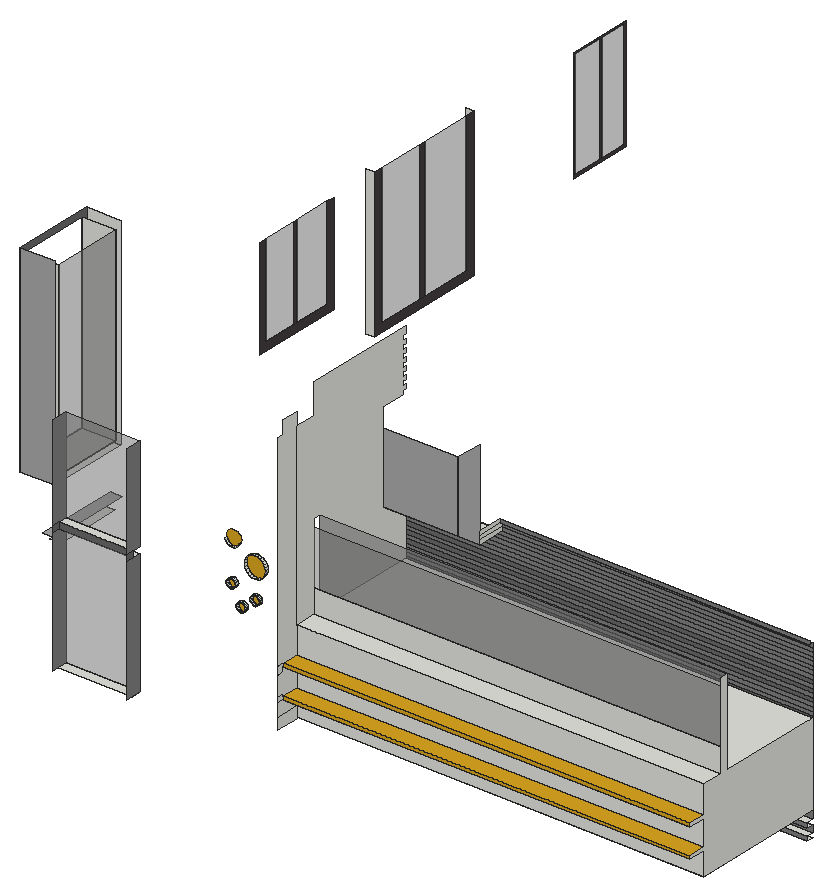
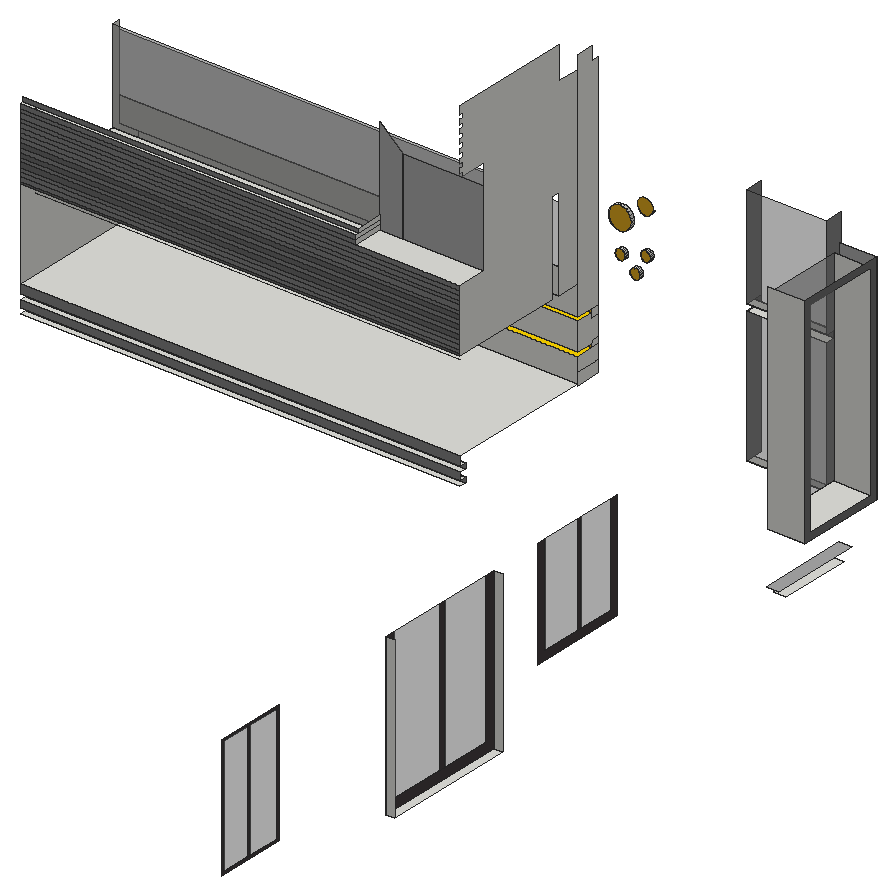
# SketchUp Ruby script. Lengths in inches.
U = 1.inch
M = Sketchup.active_model
def pt(a) = Geom::Point3d.new(a.map { |v| v * U })
def face(e, loops, mat)
  f = e.add_face(loops[0].map { |a| pt(a) })
  loops[1..].each { |l| e.add_face(l.map { |a| pt(a) }).erase! }
  f.material = f.back_material = mat if mat
  f
end
# faces: each face lists its corners as indices into pts; further lists are holes
def faces(e, pts, list, mat = nil) = list.each { |f| face(e, (f[0].is_a?(Array) ? f : [f]).map { |l| l.map { |i| pts[i] } }, mat) }
# xy, xz, yz: faces in a plane at the given z, y or x. An outline is a flat list of corners, or four numbers for a rectangle; further outlines are holes
def ring(l) = l.size == 4 ? [[l[0], l[1]], [l[2], l[1]], [l[2], l[3]], [l[0], l[3]]] : l.each_slice(2).to_a
def flat(e, list, mat, &to3) = list.each { |f| face(e, (f[0].is_a?(Array) ? f : [f]).map { |l| ring(l).map { |u, v| to3.(u, v) } }, mat) }
def xy(e, z, list, mat = nil) = flat(e, list, mat) { |x, y| [x, y, z] }
def xz(e, y, list, mat = nil) = flat(e, list, mat) { |x, z| [x, y, z] }
def yz(e, x, list, mat = nil) = flat(e, list, mat) { |y, z| [x, y, z] }
def lines(e, pts, list) = list.each { |a, b| e.add_line(pt(pts[a]), pt(pts[b])) }
# prism: a flat outline (further loops are holes) pulled along v
def prism(e, loops, v, mat = nil)
  f = face(e, loops, mat); d = Geom::Vector3d.new(v.map { |x| x * U })
  f.pushpull(f.normal.samedirection?(d) ? d.length : -d.length)
end
def box(e, o, s, mat = nil) = prism(e, [[o, [o[0] + s[0], o[1], o[2]], [o[0] + s[0], o[1] + s[1], o[2]], [o[0], o[1] + s[1], o[2]]]], [0, 0, s[2]], mat)
def at(x, y, z, deg = 0) = Geom::Transformation.translation(pt([x, y, z])) * Geom::Transformation.rotation(ORIGIN, Z_AXIS, deg.degrees)
def axes(o, x, y, z) = Geom::Transformation.new([*x, 0, *y, 0, *z, 0, *pt(o).to_a, 1])
def part(name) = M.definitions.add(name)
# library, detail: a bought-in or finely detailed component or shape, given as its bounding box
def library(name, o, s) = part(name).tap { |d| box(d.entities, o, s) }
def detail(e, o, s) = box(e.add_group.entities, o, s)
def put(e, d, t, mat = nil) = e.add_instance(d, t).tap { |i| i.material = mat if mat }
def group(e, t, mat = nil) = e.add_group.tap { |g| g.transformation = t; g.material = mat if mat }.entities
root = M.entities
M.materials.add("[0045_Goldenrod]").color = [218, 165, 32]
M.materials.add("[0046_Gold]").color = [255, 215, 0]
M.materials.add("[0132_LightGray]").color = [169, 169, 169]
M.materials.add("[0133_Gray]").color = [128, 128, 128]
M.materials.add("[0134_DimGray]").color = [105, 105, 105]
M.materials.add("[Asphalt New]").color = [67, 60, 62]
M.materials.add("[Translucent Glass Gray]").color = [128, 128, 128]
M.materials["[Translucent Glass Gray]"].alpha = 0.5
xy(root,66.12,[[241.18,136.58,366.5,138.52]])
xy(root,67.4375,[[174.32,88.83,197.1,91.46]])
xy(root,67.625,[[241.18,136.58,366.5,138.52]])
xy(root,69.69,[[241.18,136.58,366.5,138.52]])
xy(root,71.22,[[241.18,136.58,366.5,138.52]])
xy(root,73.87,[[241.18,96.65,366.5,138.52]])
xy(root,75.79,[[142.375,125.2,145.875,145.94]])
xy(root,78.39,[[142.375,122.6,145.875,148.54]],"[0132_LightGray]")
xy(root,79.7,[[143.25,245.77,145.875,284.1]])
xy(root,80.87,[[241.18,91.46,366.5,96.65]],"[0046_Gold]")
xy(root,81.9375,[[241.18,91.46,366.5,96.65]],"[0045_Goldenrod]")
xy(root,89.85,[[241.18,91.46,366.5,96.65]],"[0046_Gold]")
xy(root,90.9375,[[241.18,91.46,366.5,96.65]],"[0045_Goldenrod]")
xy(root,92.89,[[135.375,122.53,145.875,148.03]])
xy(root,94.72,[[135.375,124.36,145.875,146.21]])
xy(root,99.3125,[[241.18,96.65,366.5,103.28],[241.18,105.72,366.5,138.52]])
xy(root,105.6875,[[174.32,88.83,197.1,91.46]])
xy(root,107.62,[[174.32,88.83,197.1,91.46]])
xy(root,117.32,[[264.37,129.83,264.37,129.9,241.18,129.9,241.18,138.52,271.01,138.52,271.01,129.83]])
xy(root,119.82,[[271.01,137.46,362.29,138.52],[362.29,137.46,366.5,138.52]])
xz(root,88.83,[[174.32,105.6875,197.1,107.62]],"[0134_DimGray]")
xz(root,90.15,[[227.13,118.98,227.72,119.06,228.26,119.28,228.72,119.64,229.08,120.11,229.31,120.65,229.38,121.23,229.31,121.8125,229.08,122.36,228.72,122.82,228.26,123.18,227.72,123.4,227.13,123.48,226.55,123.4,226.01,123.18,225.54,122.82,225.19,122.36,224.96,121.8125,224.88,121.23,224.96,120.65,225.19,120.11,225.54,119.64,226.01,119.28,226.55,119.06]],"[0045_Goldenrod]")
xz(root,90.27,[[234.1875,112.62,235.03,112.73,235.8125,113.05,236.49,113.57,237,114.24,237.33,115.02,237.4375,115.87,237.33,116.71,237,117.49,236.49,118.16,235.8125,118.68,235.03,119.01,234.1875,119.12,233.35,119.01,232.5625,118.68,231.89,118.16,231.375,117.49,231.05,116.71,230.9375,115.87,231.05,115.02,231.375,114.24,231.89,113.57,232.5625,113.05,233.35,112.73]],"[0045_Goldenrod]")
xz(root,90.33,[[234.12,105.15,234.49,105.2,234.84,105.34,235.13,105.57,235.36,105.87,235.5,106.21,235.55,106.59,235.5,106.96,235.36,107.3,235.13,107.6,234.84,107.83,234.49,107.97,234.12,108.02,233.74,107.97,233.4,107.83,233.1,107.6,232.87,107.3,232.73,106.96,232.68,106.59,232.73,106.21,232.87,105.87,233.1,105.57,233.4,105.34,233.74,105.2]],"[0045_Goldenrod]")
xz(root,90.4,[[229.8,101.75,230.17,101.79,230.51,101.9375,230.8125,102.17,231.04,102.46,231.18,102.8125,231.23,103.18,231.18,103.55,231.04,103.9,230.8125,104.2,230.51,104.43,230.17,104.57,229.8,104.62,229.42,104.57,229.08,104.43,228.78,104.2,228.55,103.9,228.41,103.55,228.36,103.18,228.41,102.8125,228.55,102.46,228.78,102.17,229.08,101.9375,229.42,101.79]],"[0045_Goldenrod]")
xz(root,90.46,[[226.74,107.31,227.11,107.35,227.46,107.5,227.75,107.73,227.98,108.02,228.125,108.37,228.18,108.74,228.125,109.12,227.98,109.46,227.75,109.76,227.46,109.99,227.11,110.13,226.74,110.18,226.37,110.13,226.02,109.99,225.72,109.76,225.49,109.46,225.35,109.12,225.3,108.74,225.35,108.37,225.49,108.02,225.72,107.73,226.02,107.5,226.37,107.35]],"[0045_Goldenrod]")
xz(root,91.46,[[241.18,80.87,366.5,81.9375],[241.18,89.85,366.5,90.9375]],"[0045_Goldenrod]")
xz(root,91.46,[[174.32,67.4375,197.1,105.6875],[174.32,107.62,197.1,136.72]],"[Translucent Glass Gray]")
xz(root,96.65,[[241.18,73.87,366.5,80.87],[241.18,81.9375,366.5,89.85],[241.18,90.9375,366.5,99.3125]])
xz(root,103.28,[[241.18,99.3125,366.5,106.59]])
xz(root,103.28,[[241.18,106.59,366.5,123.39]],"[Translucent Glass Gray]")
xz(root,105.72,[[241.18,99.3125,366.5,125.6875]],"[Translucent Glass Gray]")
xz(root,122.53,[[135.375,92.89,145.875,154.77]],"[0132_LightGray]")
xz(root,124.36,[[135.375,94.72,145.875,152.9375]])
xz(root,129.83,[[264.37,117.32,271.01,117.32,271.01,144.82,264.37,139.03]],"[0132_LightGray]")
xz(root,129.9,[[241.18,117.32,264.37,139.03]],"[0132_LightGray]")
xz(root,136.58,[[241.18,66.12,366.5,67.625],[241.18,69.69,366.5,71.22]],"[0133_Gray]")
xz(root,137.46,[[271.01,119.82,366.5,121]],"[0133_Gray]")
xz(root,138.52,[[241.18,67.625,366.5,69.69],[241.18,71.22,366.5,73.87],[241.18,99.82,366.5,101],[241.18,101,366.5,102.32],[241.18,102.32,366.5,103.5],
  [241.18,104.82,366.5,106],[241.18,107.32,366.5,108.5],[241.18,109.82,366.5,111],[241.18,111,366.5,112.32],[241.18,112.32,366.5,113.5],
  [241.18,113.5,366.5,114.82],[241.18,114.82,366.5,116],[241.18,116,366.5,117.32],[271.01,117.32,366.5,118.5],[271.01,118.5,366.5,119.82]],"[0133_Gray]")
xz(root,138.52,[[241.18,99.3125,366.5,99.82],[241.18,103.5,366.5,104.82],[241.18,106,366.5,107.32],[241.18,108.5,366.5,109.82]],"[0134_DimGray]")
xz(root,146.21,[[135.375,94.72,145.875,152.9375]])
xz(root,148.03,[[135.375,92.89,145.875,154.77]])
xz(root,245.77,[[143.25,79.7,145.875,125.14]])
xz(root,284.1,[[143.25,79.7,145.875,125.14]])
yz(root,135.375,[[[122.53,92.89,148.03,154.77],[124.36,94.72,146.21,152.9375]]],"[0134_DimGray]")
yz(root,145.875,[[245.77,79.7,245.77,125.14,248.5,125.14,248.5,82.42,281.37,82.42,281.37,125.14,284.1,125.14,284.1,79.7],[263.24,82.42,264.94,125.14],[[322.32,89.76,342.57,124.57],[323.02,90.45,341.875,123.87]],[332.45,90.45,333.16,123.87],[201.67,94.21,201.67,125.14,204.1,125.14,204.1,96.64,227.54,96.64,227.54,125.14,229.97,125.14,229.97,94.21],
  [214.54,96.64,215.82,125.14]],"[Asphalt New]")
yz(root,145.875,[[248.5,82.42,263.24,125.14],[264.94,82.42,281.37,125.14],[323.02,90.45,332.45,123.87],[333.16,90.45,341.875,123.87],[124.36,94.72,146.21,152.9375],
  [204.1,96.64,214.54,125.14],[215.82,96.64,227.54,125.14]],"[Translucent Glass Gray]")
yz(root,174.32,[[86.4,67.4375,91.46,105.6875],[86.4,107.62,91.46,136.72]],"[0133_Gray]")
yz(root,174.32,[[86.4,105.6875,88.83,107.62]],"[0134_DimGray]")
yz(root,197.1,[[86.4,67.4375,91.46,105.6875],[86.4,107.62,91.46,136.72]],"[0133_Gray]")
yz(root,197.1,[[86.4,105.6875,88.83,107.62]],"[0134_DimGray]")
yz(root,241.18,[[89.33,73.43,96.65,76.93],[89.33,76.93,96.65,80.87],[89.33,80.87,91.46,82.5625],[91.46,81.9375,96.65,81.9375,96.65,89.85,91.46,89.85,91.46,88.48,89.33,88.48,89.33,82.5625,91.46,82.5625],[89.33,88.48,91.46,90.9375],
  [89.33,90.9375,96.65,90.9375,96.65,158,91.46,158,91.46,154.0625,89.33,154.0625],[96.65,99.3125,103.28,99.3125,103.28,125.6875,105.72,125.6875,105.72,99.3125,138.52,99.3125,138.52,117.32,129.9,117.32,129.9,144.82,137.46,144.82,137.46,146,138.52,146,138.52,147.32,137.46,147.32,137.46,148.5,138.52,148.5,138.52,149.82,137.46,149.82,137.46,151,138.52,151,138.52,152.32,137.46,152.32,137.46,153.5,138.52,153.5,138.52,154.82,137.46,154.82,137.46,156,138.52,156,138.52,157.32,137.46,157.32,137.46,158.5,138.52,158.5,138.52,159.82,137.46,159.82,137.46,161.04,138.52,161.04,138.52,163.35,103.2,163.35,103.2,154.0625,96.65,154.0625]])
yz(root,264.37,[[129.83,117.32,129.9,139.03]])
yz(root,271.01,[[129.83,117.32,138.52,118.5],[129.83,118.5,138.52,119.82],[129.83,119.82,137.46,121]])
yz(root,366.5,[[96.65,73.87,138.52,73.87,138.52,99.3125,105.72,99.3125,105.72,125.6875,103.28,125.6875,103.28,99.3125,96.65,99.3125,96.65,90.9375,91.46,90.9375,91.46,89.85,96.65,89.85,96.65,81.9375,91.46,81.9375,91.46,80.87,96.65,80.87]])
p = [[229.42,89.33,101.79],[229.8,89.33,101.75],[229.8,90.4,101.75],[229.42,90.4,101.79],[230.17,89.33,101.79],[230.17,90.4,101.79],
  [229.08,89.33,101.9375],[229.08,90.4,101.9375],[230.51,89.33,101.9375],[230.51,90.4,101.9375],[228.78,89.33,102.17],[228.78,90.4,102.17],
  [230.8125,89.33,102.17],[230.8125,90.4,102.17],[228.55,89.33,102.46],[228.55,90.4,102.46],[231.04,89.33,102.46],[231.04,90.4,102.46],
  [228.41,89.33,102.8125],[228.41,90.4,102.8125],[231.18,89.33,102.8125],[231.18,90.4,102.8125],[228.36,89.33,103.18],[228.36,90.4,103.18],
  [231.23,89.33,103.18],[231.23,90.4,103.18],[228.41,89.33,103.55],[228.41,90.4,103.55],[231.18,89.33,103.55],[231.18,90.4,103.55],
  [228.55,89.33,103.9],[228.55,90.4,103.9],[231.04,89.33,103.9],[231.04,90.4,103.9],[228.78,89.33,104.2],[228.78,90.4,104.2],
  [230.8125,89.33,104.2],[230.8125,90.4,104.2],[229.08,89.33,104.43],[229.08,90.4,104.43],[230.51,89.33,104.43],[230.51,90.4,104.43],
  [229.42,89.33,104.57],[229.42,90.4,104.57],[230.17,89.33,104.57],[230.17,90.4,104.57],[229.8,89.33,104.62],[229.8,90.4,104.62],
  [233.74,89.33,105.2],[234.12,89.33,105.15],[234.12,90.33,105.15],[233.74,90.33,105.2],[234.49,89.33,105.2],[234.49,90.33,105.2],
  [233.4,89.33,105.34],[233.4,90.33,105.34],[234.84,89.33,105.34],[234.84,90.33,105.34],[233.1,89.33,105.57],[233.1,90.33,105.57],
  [235.13,89.33,105.57],[235.13,90.33,105.57],[232.87,89.33,105.87],[232.87,90.33,105.87],[235.36,89.33,105.87],[235.36,90.33,105.87],
  [232.73,89.33,106.21],[232.73,90.33,106.21],[235.5,89.33,106.21],[235.5,90.33,106.21],[232.68,89.33,106.59],[232.68,90.33,106.59],
  [235.55,89.33,106.59],[235.55,90.33,106.59],[232.73,89.33,106.96],[232.73,90.33,106.96],[235.5,89.33,106.96],[235.5,90.33,106.96],
  [232.87,89.33,107.3],[232.87,90.33,107.3],[235.36,89.33,107.3],[235.36,90.33,107.3],[226.37,89.33,107.35],[226.74,89.33,107.31],
  [226.74,90.46,107.31],[226.37,90.46,107.35],[227.11,89.33,107.35],[227.11,90.46,107.35],[233.1,89.33,107.6],[233.1,90.33,107.6],
  [235.13,89.33,107.6],[235.13,90.33,107.6],[226.02,89.33,107.5],[226.02,90.46,107.5],[227.46,89.33,107.5],[227.46,90.46,107.5],
  [225.72,89.33,107.73],[225.72,90.46,107.73],[227.75,89.33,107.73],[227.75,90.46,107.73],[233.4,89.33,107.83],[233.4,90.33,107.83],
  [234.84,89.33,107.83],[234.84,90.33,107.83],[225.49,89.33,108.02],[225.49,90.46,108.02],[227.98,89.33,108.02],[227.98,90.46,108.02],
  [233.74,89.33,107.97],[233.74,90.33,107.97],[234.49,89.33,107.97],[234.49,90.33,107.97],[225.35,89.33,108.37],[225.35,90.46,108.37],
  [228.125,89.33,108.37],[228.125,90.46,108.37],[234.12,89.33,108.02],[234.12,90.33,108.02],[225.3,89.33,108.74],[225.3,90.46,108.74],
  [228.18,89.33,108.74],[228.18,90.46,108.74],[225.35,89.33,109.12],[225.35,90.46,109.12],[228.125,89.33,109.12],[228.125,90.46,109.12],
  [225.49,89.33,109.46],[225.49,90.46,109.46],[227.98,89.33,109.46],[227.98,90.46,109.46],[225.72,89.33,109.76],[225.72,90.46,109.76],
  [227.75,89.33,109.76],[227.75,90.46,109.76],[226.02,89.33,109.99],[226.02,90.46,109.99],[227.46,89.33,109.99],[227.46,90.46,109.99],
  [226.37,89.33,110.13],[226.37,90.46,110.13],[227.11,89.33,110.13],[227.11,90.46,110.13],[226.74,89.33,110.18],[226.74,90.46,110.18],
  [233.35,89.33,112.73],[234.1875,89.33,112.62],[234.1875,90.27,112.62],[233.35,90.27,112.73],[235.03,89.33,112.73],[235.03,90.27,112.73],
  [232.5625,89.33,113.05],[232.5625,90.27,113.05],[235.8125,89.33,113.05],[235.8125,90.27,113.05],[231.89,89.33,113.57],[231.89,90.27,113.57],
  [236.49,89.33,113.57],[236.49,90.27,113.57],[231.375,89.33,114.24],[231.375,90.27,114.24],[237,89.33,114.24],[237,90.27,114.24],
  [231.05,89.33,115.02],[231.05,90.27,115.02],[237.33,89.33,115.02],[237.33,90.27,115.02],[230.9375,89.33,115.87],[230.9375,90.27,115.87],
  [237.4375,89.33,115.87],[237.4375,90.27,115.87],[231.05,89.33,116.71],[231.05,90.27,116.71],[237.33,89.33,116.71],[237.33,90.27,116.71],
  [231.375,89.33,117.49],[231.375,90.27,117.49],[237,89.33,117.49],[237,90.27,117.49],[231.89,89.33,118.16],[231.89,90.27,118.16],
  [236.49,89.33,118.16],[236.49,90.27,118.16],[232.5625,89.33,118.68],[232.5625,90.27,118.68],[235.8125,89.33,118.68],[235.8125,90.27,118.68],
  [233.35,89.33,119.01],[233.35,90.27,119.01],[235.03,89.33,119.01],[235.03,90.27,119.01],[226.55,89.33,119.06],[227.13,89.33,118.98],
  [227.13,90.15,118.98],[226.55,90.15,119.06],[227.72,89.33,119.06],[227.72,90.15,119.06],[234.1875,89.33,119.12],[234.1875,90.27,119.12],
  [226.01,89.33,119.28],[226.01,90.15,119.28],[228.26,89.33,119.28],[228.26,90.15,119.28],[225.54,89.33,119.64],[225.54,90.15,119.64],
  [228.72,89.33,119.64],[228.72,90.15,119.64],[225.19,89.33,120.11],[225.19,90.15,120.11],[229.08,89.33,120.11],[229.08,90.15,120.11],
  [224.96,89.33,120.65],[224.96,90.15,120.65],[229.31,89.33,120.65],[229.31,90.15,120.65],[362.29,138.52,98.5],[241.18,138.52,98.5]]
faces(root,p,[[0,1,2,3],[1,4,5,2],[6,0,3,7],[4,8,9,5],[10,6,7,11],[8,12,13,9],[14,10,11,15],[12,16,17,13],
  [18,14,15,19],[16,20,21,17],[22,18,19,23],[20,24,25,21],[26,22,23,27],[24,28,29,25],[30,26,27,31],[28,32,33,29],
  [34,30,31,35],[32,36,37,33],[38,34,35,39],[36,40,41,37],[42,38,39,43],[40,44,45,41],[46,42,43,47],[44,46,47,45],
  [48,49,50,51],[49,52,53,50],[54,48,51,55],[52,56,57,53],[58,54,55,59],[56,60,61,57],[62,58,59,63],[60,64,65,61],
  [66,62,63,67],[64,68,69,65],[70,66,67,71],[68,72,73,69],[74,70,71,75],[72,76,77,73],[78,74,75,79],[76,80,81,77],
  [82,83,84,85],[83,86,87,84],[88,78,79,89],[80,90,91,81],[92,82,85,93],[86,94,95,87],[96,92,93,97],[94,98,99,95],
  [100,88,89,101],[90,102,103,91],[104,96,97,105],[98,106,107,99],[108,100,101,109],[102,110,111,103],[112,104,105,113],[106,114,115,107],
  [116,108,109,117],[110,116,117,111],[118,112,113,119],[114,120,121,115],[122,118,119,123],[120,124,125,121],[126,122,123,127],[124,128,129,125],
  [130,126,127,131],[128,132,133,129],[134,130,131,135],[132,136,137,133],[138,134,135,139],[136,140,141,137],[142,138,139,143],[140,142,143,141],
  [144,145,146,147],[145,148,149,146],[150,144,147,151],[148,152,153,149],[154,150,151,155],[152,156,157,153],[158,154,155,159],[156,160,161,157],
  [162,158,159,163],[160,164,165,161],[166,162,163,167],[164,168,169,165],[170,166,167,171],[168,172,173,169],[174,170,171,175],[172,176,177,173],
  [178,174,175,179],[176,180,181,177],[182,178,179,183],[180,184,185,181],[186,182,183,187],[184,188,189,185],[190,191,192,193],[191,194,195,192],
  [196,186,187,197],[188,196,197,189],[198,190,193,199],[194,200,201,195],[202,198,199,203],[200,204,205,201],[206,202,203,207],[204,208,209,205],
  [210,206,207,211],[208,212,213,209]])
lines(root,p,[[214,215]])
